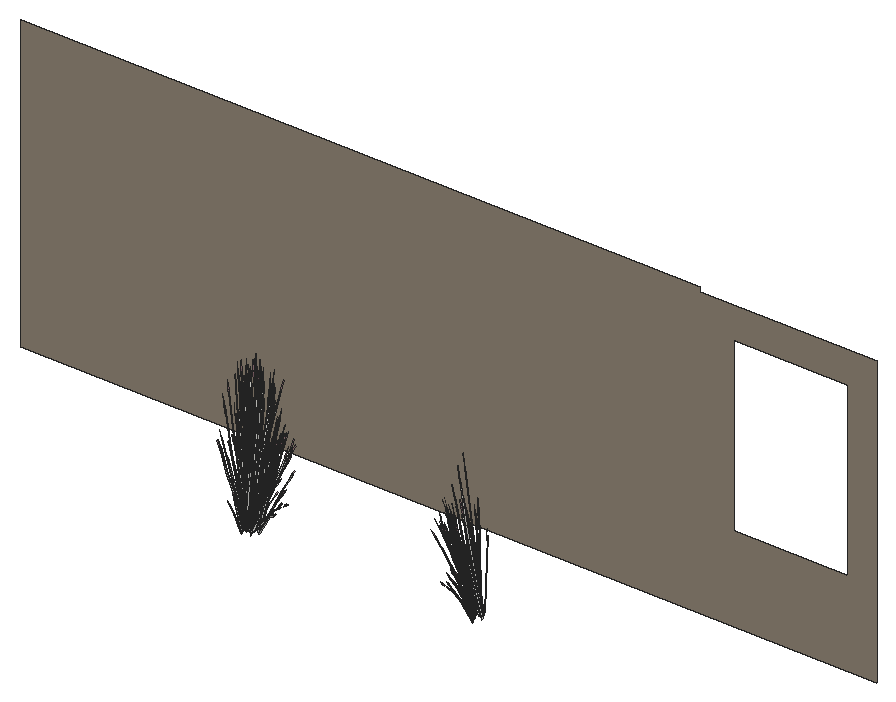
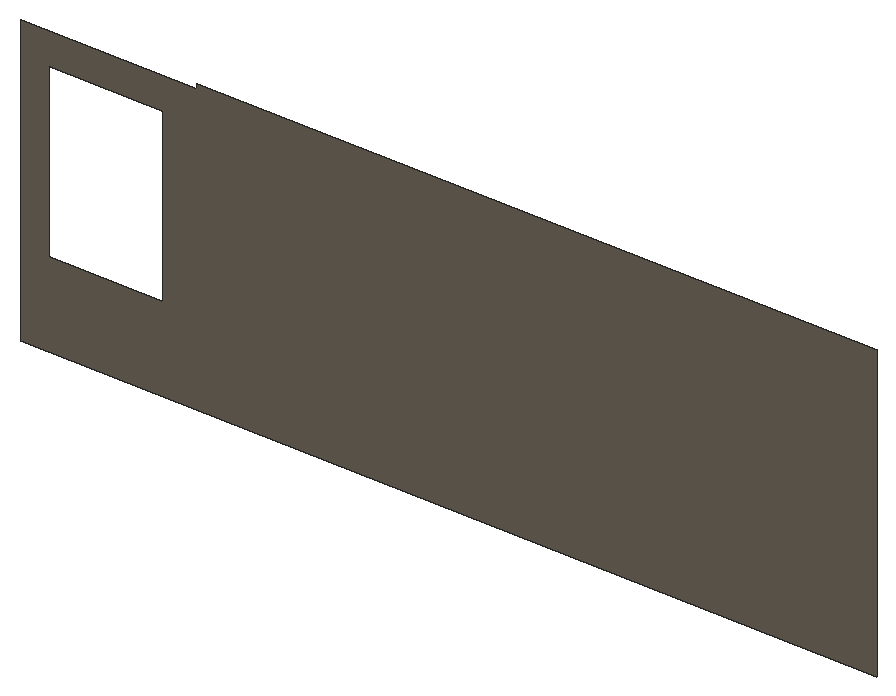
# SketchUp Ruby script. Lengths in inches.
U = 1.inch
M = Sketchup.active_model
def pt(a) = Geom::Point3d.new(a.map { |v| v * U })
def face(e, loops, mat)
  f = e.add_face(loops[0].map { |a| pt(a) })
  loops[1..].each { |l| e.add_face(l.map { |a| pt(a) }).erase! }
  f.material = f.back_material = mat if mat
  f
end
# faces: each face lists its corners as indices into pts; further lists are holes
def faces(e, pts, list, mat = nil) = list.each { |f| face(e, (f[0].is_a?(Array) ? f : [f]).map { |l| l.map { |i| pts[i] } }, mat) }
# xy, xz, yz: faces in a plane at the given z, y or x. An outline is a flat list of corners, or four numbers for a rectangle; further outlines are holes
def ring(l) = l.size == 4 ? [[l[0], l[1]], [l[2], l[1]], [l[2], l[3]], [l[0], l[3]]] : l.each_slice(2).to_a
def flat(e, list, mat, &to3) = list.each { |f| face(e, (f[0].is_a?(Array) ? f : [f]).map { |l| ring(l).map { |u, v| to3.(u, v) } }, mat) }
def xy(e, z, list, mat = nil) = flat(e, list, mat) { |x, y| [x, y, z] }
def xz(e, y, list, mat = nil) = flat(e, list, mat) { |x, z| [x, y, z] }
def yz(e, x, list, mat = nil) = flat(e, list, mat) { |y, z| [x, y, z] }
def lines(e, pts, list) = list.each { |a, b| e.add_line(pt(pts[a]), pt(pts[b])) }
# prism: a flat outline (further loops are holes) pulled along v
def prism(e, loops, v, mat = nil)
  f = face(e, loops, mat); d = Geom::Vector3d.new(v.map { |x| x * U })
  f.pushpull(f.normal.samedirection?(d) ? d.length : -d.length)
end
def box(e, o, s, mat = nil) = prism(e, [[o, [o[0] + s[0], o[1], o[2]], [o[0] + s[0], o[1] + s[1], o[2]], [o[0], o[1] + s[1], o[2]]]], [0, 0, s[2]], mat)
def at(x, y, z, deg = 0) = Geom::Transformation.translation(pt([x, y, z])) * Geom::Transformation.rotation(ORIGIN, Z_AXIS, deg.degrees)
def axes(o, x, y, z) = Geom::Transformation.new([*x, 0, *y, 0, *z, 0, *pt(o).to_a, 1])
def part(name) = M.definitions.add(name)
# library, detail: a bought-in or finely detailed component or shape, given as its bounding box
def library(name, o, s) = part(name).tap { |d| box(d.entities, o, s) }
def detail(e, o, s) = box(e.add_group.entities, o, s)
def put(e, d, t, mat = nil) = e.add_instance(d, t).tap { |i| i.material = mat if mat }
def group(e, t, mat = nil) = e.add_group.tap { |g| g.transformation = t; g.material = mat if mat }.entities
root = M.entities
M.materials.add("LightPink_Translucent").color = [144, 107, 117]
M.materials["LightPink_Translucent"].alpha = 0.75
M.materials.add("Plaster_04_1K").color = [142, 132, 117]
c1 = part("blade")
p = [[2.15,0.21,22],[0,0.17,0],[0.09,0.45,0],[2.18,0.31,22],[2.29,0.31,22],[0.38,0.45,0],
  [2.48,0.24,33],[2.49,0.24,33],[2.48,0.22,33]]
faces(c1.entities,p,[[0,1,2,3],[4,5,2,3],[6,3,4,7],[8,0,3,6]])
c2 = part("seeds")
p = [[0.3,-0.1,1.38],[-0.01,-0.03,1.59],[-0.01,-0.03,0.03],[0.14,-0.07,-0.07],[0.29,-0.03,3],[0.15,0.01,3.11]]
faces(c2.entities,p,[[0,1,2,3],[1,0,4,5]],"LightPink_Translucent")
c3 = part("blade with seeds")
put(c3.entities,c1,at(0,0,0))
put(c3.entities,c2,axes([2.4,0.25,30.99],[1.5799,-0.05474,1.17369],[-0.12525,1.92788,0.29478],[-0.07173,-0.02425,1.56792]))
xz(root,63.98,[[[48,-6,408,-6,408,114.97,333.82,114.97,333.82,117,48,117],[348,30,396,102]]],"Plaster_04_1K")
put(root,c3,axes([182.11,13.09,-3.52],[0,0.61104,0.49651],[-0.85008,0,0],[0,-0.13917,1.57504]))
put(root,c3,axes([186,15.4,-3.81],[-0.46912,-0.61443,-0.05142],[0.79476,-0.34146,0.51607],[-0.19584,0.0585,1.6363]))
put(root,c3,axes([182.99,15.125,-1],[0.54391,0.41056,-0.5672],[-0.57458,0.35956,-0.43934],[-0.08276,0.2086,1.08528]))
put(root,c3,axes([185.79,15.32,-3.97],[-0.70886,-0.15119,-0.30978],[0.17848,-0.53243,0.30978],[-0.1429,0.0614,1.38974]))
put(root,c3,axes([182.75,14.82,-0.95],[0.5141,-0.32171,0.35414],[0.48666,0.36734,-0.4572],[-0.07405,0.18664,0.87481]))
put(root,c3,axes([183.97,13.23,-3.33],[-0.85568,-0.29155,-0.29095],[0.41201,-0.61537,-0.50002],[-0.02689,-0.15109,1.59708]))
put(root,c3,axes([186.19,13.05,-3.16],[-0.02076,-0.57531,1.41272],[0.93937,0.14913,0.59816],[-0.22217,0.31481,1.3335]))
put(root,c3,axes([182.42,14.91,-0.6],[0.83505,0.03027,-0.13498],[-0.02282,0.57322,-0.74919],[-0.05801,0.22077,1.13838]))
put(root,c3,axes([182.4,15.74,-3.18],[0.69024,-0.1082,0.06507],[0.15868,0.43593,-0.86304],[-0.04376,0.22067,0.7736]))
put(root,c3,axes([185.67,13.78,-3.33],[0.08854,0.69723,-0.29095],[-0.92215,0.04216,-0.50002],[-0.16238,0.09287,1.59708]))
put(root,c3,axes([183.58,12.61,-3.9],[-0.31203,-0.62659,-0.69835],[0.89884,-0.22566,-0.18329],[-0.03449,-0.21218,1.54149]))
put(root,c3,axes([185.625,10.62,-0.97],[-0.74352,0.28449,-0.1216],[-0.36538,-0.50492,-0.67495],[-0.0981,-0.21277,1.02557]))
put(root,c3,axes([184.99,10.64,-1.32],[-0.7469,-0.15318,-0.51099],[0.25601,-0.52518,-0.3958],[-0.06849,-0.21144,0.97773]))
put(root,c3,axes([183.61,14.54,-2.125],[-0.0186,-0.23452,1.71376],[0.80601,0.15558,0.13857],[-0.04985,0.33422,0.73262]))
put(root,c3,axes([182.11,12.54,-3.97],[0.53038,-0.38124,-0.30978],[0.53038,0.38124,0.30978],[0,-0.1228,1.38974]))
put(root,c3,axes([184.5,10.07,-3.87],[-0.52505,0.35054,-0.03893],[-0.48109,-0.38392,-0.17649],[-0.03387,-0.10878,0.58215]))
put(root,c3,axes([184.29,13.53,-3.64],[0.96033,0.12874,0.45755],[-0.19544,0.7271,0.17955],[-0.14034,-0.07021,1.58856]))
put(root,c3,axes([184.04,13.4,-3.28],[-0.36864,0.55059,0.44739],[-0.76598,-0.26498,-0.21531],[0,-0.12692,1.43643]))
put(root,c3,axes([185.26,10.74,-1.02],[-0.36264,-0.49684,-0.71045],[0.74649,-0.27689,0.08574],[-0.0848,-0.24006,1.00501]))
put(root,c3,axes([183.78,14.6875,-3.53],[0.81646,-0.16218,0.17642],[0.20161,0.60355,0.35086],[-0.07282,-0.08794,1.60407]))
put(root,c3,axes([184.83,14.78,-3.8],[-0.76598,-0.27433,0],[0.36864,-0.57001,0],[0,0,1.62707]))
put(root,c3,axes([185.4,10.82,-0.95],[-0.22906,0.4699,0.35414],[-0.66828,-0.13705,-0.4572],[-0.06128,-0.18919,0.87481]))
put(root,c3,axes([186.6,15.47,-3.625],[0.47504,0.61229,0],[-0.79476,0.34146,-0.51607],[-0.18101,0.07777,1.63711]))
put(root,c3,axes([184.18,15.73,-0.9375],[-0.74868,-0.15974,0.53283],[0.25601,-0.52518,0.43934],[0.04499,0.20653,1.10256]))
put(root,c3,axes([183.98,15.77,-1.27],[-0.55987,0.20767,0.0643],[-0.27403,-0.37869,0.50621],[0.05407,0.16693,0.77189]))
put(root,c3,axes([186.21,14.72,-3.53],[0.21949,-0.60727,0.17642],[0.8032,0.17185,0.35086],[-0.13875,0.00296,1.60407]))
put(root,c3,axes([185.83,13.92,-3.38],[0.56134,0.36712,0.1448],[-0.46823,0.41419,-0.41347],[-0.13033,0.05599,1.26744]))
put(root,c3,axes([185.64,13.46,-3.7],[-0.70674,-0.52593,-0.06131],[0.70717,-0.52625,0],[-0.02468,-0.01837,1.75571]))
put(root,c3,axes([185.82,13.65,-3.28],[0.82508,-0.03772,0.44739],[0.07462,0.62614,-0.21531],[-0.14771,0.06346,1.43643]))
put(root,c3,axes([186.02,15.09,-3.67],[0.95122,0.19861,0.30756],[-0.23797,0.7099,-0.36492],[-0.15744,0.08885,1.64885]))
put(root,c3,axes([184.63,9.64,-4.51],[-0.12744,0.02202,1.76342],[-0.70477,-0.24781,-0.26939],[0.01183,-0.2067,0.30037]))
put(root,c3,axes([186.43,15.05,-3.52],[0.7111,-0.30552,0.49651],[0.42504,0.54784,0],[-0.16196,0.06958,1.57504]))
put(root,c3,axes([185.33,10.32,-1.47],[0.22906,-0.4699,-0.35414],[0.66828,0.13705,0.4572],[-0.06128,-0.18919,0.87481]))
put(root,c3,axes([184.21,12.86,-3.64],[0.33034,0.68327,0.45755],[-0.94388,0.2376,0.17955],[0.01154,-0.12555,1.58856]))
put(root,c3,axes([184.06,12.77,-3.79],[0.36864,-0.55059,-0.44739],[0.76598,0.26498,0.21531],[0,-0.12692,1.43643]))
put(root,c3,axes([185,14.55,-3.8],[-0.24791,-0.5268,0],[0.70791,-0.18448,0],[0,0,1.54371]))
put(root,c3,axes([184.1,15.66,-4.51],[0.12297,-0.03325,1.76342],[0.73967,0.18301,-0.26939],[0.02163,0.20626,0.30037]))
put(root,c3,axes([184.26,15.84,-1.47],[-0.22906,0.4699,-0.35414],[-0.66828,-0.13705,0.4572],[0.06128,0.18919,0.87481]))
put(root,c3,axes([186,13.51,-3.79],[-0.36864,0.55059,-0.44739],[-0.76598,-0.26498,0.21531],[0,0.12692,1.43643]))
put(root,c3,axes([185.61,10.39,-1.27],[0.55987,-0.20767,0.0643],[0.27403,0.37869,0.50621],[-0.05407,-0.16693,0.77189]))
put(root,c3,axes([183.79,16.68,-1.28],[0.09631,0.0984,1.74944],[0.77725,0.03866,-0.27667],[0.07816,0.217,0.14031]))
put(root,c3,axes([187.46,13.17,-3.53],[-0.59697,-0.44509,0.17642],[0.60159,-0.4317,0.35086],[-0.06593,0.0909,1.60407]))
put(root,c3,axes([185.4,12.92,-3.79],[0,-0.70701,0],[0.95008,0,0],[0,0,1.79456]))
put(root,c3,axes([185.41,10.43,-1.27],[0.74868,0.15974,0.48003],[-0.25601,0.52518,0.3958],[-0.04499,-0.20653,0.9933]))
put(root,c3,axes([184.51,13.04,-3.57],[0.8561,0.29616,0.24065],[-0.41201,0.61537,0.50002],[0,-0.14185,1.60543]))
put(root,c3,axes([185.875,13.2,-3.71],[0,0.70667,-0.05637],[-0.95008,0,0],[0,0.02221,1.79368]))
put(root,c3,axes([184.24,12.63,-3.28],[-0.82508,0.03772,0.44739],[-0.07462,-0.62614,-0.21531],[0.14771,-0.06346,1.43643]))
put(root,c3,axes([184.19,15.35,-0.95],[0.22906,-0.4699,0.35414],[0.66828,0.13705,-0.4572],[0.06128,0.18919,0.87481]))
put(root,c3,axes([183.85,11.56,-3.53],[-0.21949,0.60727,0.17642],[-0.8032,-0.17185,0.35086],[0.13875,-0.00296,1.60407]))
put(root,c3,axes([185.42,14.57,-3.71],[0.33034,0.70197,-0.06012],[-0.94388,0.24598,0],[0.01154,0.02451,1.72173]))
put(root,c3,axes([183.46,10.81,-3.625],[-0.47504,-0.61229,0],[0.79476,-0.34146,-0.51607],[0.18101,-0.07777,1.63711]))
put(root,c3,axes([184.33,15.42,-1.02],[0.36264,0.49684,-0.71045],[-0.74649,0.27689,0.08574],[0.0848,0.24006,1.00501]))
put(root,c3,axes([188.15,13.64,-3.8],[-0.94962,-0.00489,-0.04976],[0,-0.68292,0.49943],[-0.02984,0.15546,1.58352]))
put(root,c3,axes([186.28,11.59,-3.53],[-0.81646,0.16218,0.17642],[-0.20161,-0.60355,0.35086],[0.07282,0.08794,1.60407]))
put(root,c3,axes([185.45,9.33,-3.23],[0.09747,0.35631,1.1486],[-0.54071,-0.19735,0.84392],[0.05818,-0.18244,0.25299]))
put(root,c3,axes([185.09,17.03,-0.35],[0.52505,-0.35054,-0.06488],[0.48109,0.38392,-0.29416],[0.03387,0.10878,0.97024]))
put(root,c3,axes([184.95,12.47,-3.64],[-0.62999,0.55453,0.45755],[-0.74845,-0.4895,0.17955],[0.15188,-0.05534,1.58856]))
put(root,c3,axes([186.02,13.34,-3.79],[0.53038,0.39469,0],[-0.53038,0.39469,0],[0,0,1.69266]))
put(root,c3,axes([186.02,12.88,-3.28],[0.36864,-0.55059,0.44739],[0.76598,0.26498,-0.21531],[0,0.12692,1.43643]))
put(root,c3,axes([185.7,14.8,-3.8],[0.76598,0.27433,0],[-0.36864,0.57001,0],[0,0,1.74954]))
put(root,c3,axes([184.6,15.52,-1.32],[0.7469,0.15318,-0.51099],[-0.25601,0.52518,-0.3958],[0.06849,0.21144,0.97773]))
put(root,c3,axes([183.97,15.55,-0.97],[0.74352,-0.28449,-0.1216],[0.36538,0.50492,-0.67495],[0.0981,0.21277,1.02557]))
put(root,c3,axes([185.77,12.75,-3.62],[-0.96033,-0.12874,0.49198],[0.19544,-0.7271,0.19306],[0.14034,0.07021,1.70813]))
put(root,c3,axes([187.76,9.91,-1.29],[-0.07716,0.04667,1.77383],[-0.75601,-0.15746,-0.16761],[-0.02737,-0.20368,0.31391]))
put(root,c3,axes([187.17,11.26,-0.97],[-0.83505,-0.03027,-0.1216],[0.02282,-0.57322,-0.67495],[0.05801,-0.22077,1.02557]))
put(root,c3,axes([187.95,13.74,-3.97],[-0.53038,0.38124,-0.30978],[-0.53038,-0.38124,0.30978],[0,0.1228,1.38974]))
put(root,c3,axes([186.4375,13.67,-3.91],[0.2786,0.55945,-0.69212],[-0.80253,0.20149,-0.18165],[0.03079,0.18945,1.52773]))
put(root,c3,axes([186.04,13.07,-3.79],[0.85008,0,0],[0,0.63259,0],[0,0,1.78407]))
put(root,c3,axes([186.84,11.35,-0.95],[-0.5141,0.32171,0.35414],[-0.48666,-0.36734,-0.4572],[0.07405,-0.18664,0.87481]))
put(root,c3,axes([185.22,12.375,-3.28],[-0.45644,-0.51287,0.44739],[0.69137,-0.36116,-0.21531],[0.14771,0.06346,1.43643]))
put(root,c3,axes([184.39,12.5,-3.33],[-0.08854,-0.69723,-0.29095],[0.92215,-0.04216,-0.50002],[0.16238,-0.09287,1.59708]))
put(root,c3,axes([186.34,13.01,-3.38],[0.70791,-0.1782,0.1448],[0.24791,0.50885,-0.41347],[0,0.11199,1.26744]))
put(root,c3,axes([186.6,11.04,-1.32],[-0.54391,-0.41056,-0.51099],[0.57458,-0.35956,-0.3958],[0.08276,-0.2086,0.97773]))
put(root,c3,axes([186.09,13.05,-3.33],[0.85568,0.29155,-0.29095],[-0.41201,0.61537,-0.50002],[0.02689,0.15109,1.59708]))
put(root,c3,axes([184.27,10.95,-3.97],[0.70886,0.15119,-0.30978],[-0.17848,0.53243,0.30978],[0.1429,-0.0614,1.38974]))
put(root,c3,axes([186.24,10.3125,-3.41],[-0.21597,0.12368,1.43002],[-0.64681,-0.21647,-0.30754],[0.1199,-0.26922,0.61141]))
put(root,c3,axes([187.95,13.19,-3.52],[0,-0.61104,0.49651],[0.85008,0,0],[0,0.13917,1.57504]))
put(root,c3,axes([188.32,13.76,-3.98],[0,0.61104,-0.49651],[-0.85008,0,0],[0,0.13917,1.57504]))
put(root,c3,axes([186.05,15.61,-1.27],[-0.75571,0.14023,0.48003],[-0.13115,-0.55007,0.3958],[0.17773,0.16212,0.9933]))
put(root,c3,axes([184.11,10.71,-3.98],[0.7111,-0.30552,-0.49651],[0.42504,0.54784,0],[0.16196,-0.06958,1.57504]))
put(root,c3,axes([185.9,15.72,-1.27],[-0.34533,0.38816,0.0643],[-0.49176,-0.22599,0.50621],[0.15898,0.12445,0.77189]))
put(root,c3,axes([185.03,14.4375,-2.125],[-0.17368,-0.19618,1.71376],[0.80256,-0.16516,0.13857],[0.18139,0.30799,0.73262]))
put(root,c3,axes([185.53,12.23,-3.38],[0.14658,-0.54532,0.1448],[0.71613,0.09466,-0.41347],[0.13033,0.05599,1.26744]))
put(root,c3,axes([186.55,11.28,-3.52],[-0.7111,-0.30552,0.49651],[0.42504,-0.54784,0],[0.16196,0.06958,1.57504]))
put(root,c3,axes([186.77,11.23,-1.02],[0.01977,-0.56521,-0.71045],[0.83252,0.03796,0.08574],[0.08786,-0.23945,1.00501]))
put(root,c3,axes([185.93,14.47,-3.82],[0.79769,-0.20732,-0.19198],[0.2803,0.59721,0.00008],[0.08805,-0.02292,1.73897]))
put(root,c3,axes([185.79,15.27,-0.95],[-0.11735,-0.49217,0.35414],[0.67083,-0.12996,-0.4572],[0.18018,0.14104,0.87481]))
put(root,c3,axes([185.94,12.7,-3.79],[0.45644,0.51287,-0.44739],[-0.69137,0.36116,0.21531],[0.14771,0.06346,1.43643]))
put(root,c3,axes([186.25,12.44,-1.53],[-0.65655,-0.31748,1.38283],[0.69326,-0.49431,0.59665],[0.21183,0.29789,1.33663]))
put(root,c3,axes([187.11,10.89,-1.47],[0.5141,-0.32171,-0.35414],[0.48666,0.36734,0.4572],[0.07405,-0.18664,0.87481]))
put(root,c3,axes([185.14,15.96,-1.29],[0.00225,-0.07398,1.77383],[0.65113,-0.32638,-0.16761],[0.22617,0.1165,0.31391]))
put(root,c3,axes([187.31,11.05,-1.27],[0.62439,0.02847,0.0643],[-0.01712,0.42991,0.50621],[0.06534,-0.16468,0.77189]))
put(root,c3,axes([187.24,15.02,-3.23],[-0.4278,-0.1757,1.1486],[0.5524,-0.17852,0.84392],[0.14899,0.15122,0.25299]))
put(root,c3,axes([185.71,14.84,-3.41],[0.01341,-0.20255,1.43002],[0.64074,-0.22625,-0.30754],[0.1978,0.24243,0.61141]))
put(root,c3,axes([187.93,10.35,-1.28],[-0.00733,-0.12161,1.74944],[-0.61946,-0.35147,-0.27667],[0.09577,-0.21306,0.14031]))
put(root,c3,axes([184.95,11.97,-3.94],[0.51177,-0.45928,-0.62353],[0.63575,0.41646,-0.16365],[0.20507,-0.11457,1.37633]))
put(root,c3,axes([187.11,11.01,-1.27],[0.54105,0.41691,0.48003],[-0.57458,0.35956,0.3958],[0.0998,-0.1956,0.9933]))
put(root,c3,axes([187.19,11.56,-3.97],[0.17848,0.53243,-0.30978],[-0.70886,0.15119,0.30978],[0.1429,0.0614,1.38974]))
put(root,c3,axes([188.53,13.29,-3.625],[0.95008,0,0],[0,0.68292,-0.51607],[0,0.15554,1.63711]))
put(root,c3,axes([185.46,12.41,-3.33],[0.76714,-0.40567,-0.29095],[0.51013,0.57321,-0.50002],[0.18927,0.05821,1.59708]))
put(root,c3,axes([187.3,15.82,-3.33],[-0.48723,-0.01916,1.0506],[0.32177,-0.40701,0.58006],[0.19248,0.1446,0.8241]))
put(root,c3,axes([187.74,12.34,-0.95],[-0.66138,0.08733,0.35414],[-0.17464,-0.49921,-0.4572],[0.18953,-0.13408,0.87481]))
put(root,c3,axes([185.83,10.94,-2.125],[-0.14147,0.21002,1.71376],[-0.59349,-0.43464,0.13857],[0.26773,-0.27089,0.73262]))
put(root,c3,axes([185.73,15.53,-0.97],[0.45276,-0.52302,-0.1216],[0.65568,0.30132,-0.67495],[0.22792,0.14777,1.02557]))
put(root,c3,axes([183.52,12.05,-4.41],[-0.74787,0.24464,1.28929],[-0.23804,-0.70192,0.50096],[0.45924,0.01168,1.46642]))
put(root,c3,axes([188.08,12.39,-0.97],[-0.70283,-0.33692,-0.1216],[0.40491,-0.48793,-0.67495],[0.19857,-0.16961,1.02557]))
put(root,c3,axes([186.27,15.27,-1.32],[0.74975,-0.14525,-0.51099],[0.13115,0.55007,-0.3958],[0.20138,0.15763,0.97773]))
put(root,c3,axes([186.96,10.96,-3.625],[0.47504,-0.61229,0],[0.79476,0.34146,-0.51607],[0.18101,0.07777,1.63711]))
put(root,c3,axes([187.75,10.69,-4.51],[-0.11372,-0.04814,1.76342],[-0.29211,-0.53779,-0.26939],[0.19706,-0.14594,0.30037]))
put(root,c3,axes([187.13,14.61,-0.95],[-0.43232,-0.38257,0.35414],[0.49364,-0.36215,-0.4572],[0.25081,0.0551,0.87481]))
put(root,c3,axes([187.39,11.33,-3.98],[0.7111,0.30552,-0.49651],[-0.42504,0.54784,0],[0.16196,0.06958,1.57504]))
put(root,c3,axes([187.52,14.95,-1.27],[-0.03826,0.46465,0.0643],[-0.57772,-0.01274,0.50621],[0.2213,0.04862,0.77189]))
put(root,c3,axes([187.36,15.68,-4.51],[0.05536,-0.08822,1.76342],[0.69692,-0.25981,-0.26939],[0.21129,0.13447,0.30037]))
put(root,c3,axes([187.58,14.81,-1.27],[-0.56024,0.40262,0.48003],[-0.48318,-0.42758,0.3958],[0.26285,0.07427,0.9933]))
put(root,c3,axes([187.73,11.99,-1.32],[-0.19519,-0.55794,-0.51099],[0.73919,-0.0976,-0.3958],[0.21183,-0.14986,0.97773]))
put(root,c3,axes([189.03,14.87,-2.07],[-0.14542,-0.51365,-0.03492],[0.68734,-0.11809,-0.15832],[0.14353,0.03256,0.52218]))
put(root,c3,axes([187.84,13.53,-0.95],[-0.63144,-0.17046,0.35414],[0.18417,-0.49731,-0.4572],[0.25423,-0.0456,0.87481]))
put(root,c3,axes([186.35,12.5,-3.94],[0.79037,0.10018,-0.62353],[-0.16679,0.61794,-0.16365],[0.23587,0.07488,1.37633]))
put(root,c3,axes([189.72,12.86,-3.74],[-0.47106,-0.39072,-0.06488],[0.51591,-0.35801,-0.29416],[0.14618,-0.02521,0.97024]))
put(root,c3,axes([188.64,10.875,-3.23],[-0.25308,0.31105,1.1486],[-0.21753,-0.4179,0.84392],[0.20902,-0.10472,0.25299]))
put(root,c3,axes([188.34,12.26,-1.27],[0.52161,0.25698,0.0643],[-0.30368,0.36595,0.50621],[0.16723,-0.11831,0.77189]))
put(root,c3,axes([188.19,12.15,-1.27],[0.18844,0.56237,0.48003],[-0.73919,0.0976,0.3958],[0.21785,-0.13226,0.9933]))
put(root,c3,axes([186.19,13.83,-2.125],[-0.28223,-0.10528,1.71376],[0.58406,-0.44165,0.13857],[0.36402,0.19924,0.73262]))
put(root,c3,axes([189.81,12.24,-1.29],[-0.09924,-0.00464,1.77383],[-0.4121,-0.49725,-0.16761],[0.1655,-0.1635,0.31391]))
put(root,c3,axes([188.28,12.04,-1.47],[0.66138,-0.08733,-0.35414],[0.17464,0.49921,0.4572],[0.18953,-0.13408,0.87481]))
put(root,c3,axes([187.75,12.21,-1.02],[0.39688,-0.48213,-0.71045],[0.69548,0.34264,0.08574],[0.23697,-0.17468,1.00501]))
put(root,c3,axes([188.41,13.6875,-1.27],[0.27906,0.41663,0.0643],[-0.50888,0.20393,0.50621],[0.22432,-0.04024,0.77189]))
put(root,c3,axes([187.74,14.81,-1.47],[0.43232,0.38257,-0.35414],[-0.49364,0.36215,0.4572],[0.25081,0.0551,0.87481]))
put(root,c3,axes([187.25,14.85,-0.97],[0.04068,-0.62141,-0.1216],[0.77029,0.01698,-0.67495],[0.29667,0.04317,1.02557]))
put(root,c3,axes([188.11,13.7,-0.97],[-0.38229,-0.5533,-0.1216],[0.6785,-0.2719,-0.67495],[0.28593,-0.073,1.02557]))
put(root,c3,axes([188.36,13.54,-1.27],[-0.21466,0.55714,0.48003],[-0.70573,-0.19051,0.3958],[0.27753,-0.03348,0.9933]))
put(root,c3,axes([187.92,14.48,-1.28],[0.16299,-0.01033,1.74944],[0.44707,-0.47471,-0.27667],[0.28992,0.06266,0.14031]))
put(root,c3,axes([188.07,13.22,-1.32],[0.20584,-0.55581,-0.51099],[0.70573,0.19051,-0.3958],[0.28414,-0.05097,0.97773]))
put(root,c3,axes([189.85,13.58,-3.23],[-0.46945,0.10088,1.1486],[0.22097,-0.4169,0.84392],[0.24904,0.02853,0.25299]))
put(root,c3,axes([188.33,11.77,-3.41],[-0.27143,-0.0181,1.43002],[-0.27808,-0.48551,-0.30754],[0.33346,-0.13735,0.61141]))
put(root,c3,axes([188.51,13.48,-1.47],[0.63144,0.17046,-0.35414],[-0.18417,0.49731,0.4572],[0.25423,-0.0456,0.87481]))
put(root,c3,axes([187.29,14.55,-1.02],[0.75952,0.01471,-0.71045],[-0.05101,0.61953,0.08574],[0.32177,0.06538,1.00501]))
put(root,c3,axes([188.83,13.38,-4.02],[-0.48937,0.07333,1.41583],[-0.07789,-0.58369,0.08104],[0.34275,-0.08835,0.80566]))
put(root,c3,axes([189.36,13,-4.51],[-0.03971,-0.09277,1.76342],[0.27541,-0.54264,-0.26939],[0.27782,-0.00781,0.30037]))
put(root,c3,axes([189.63,15.34,-1.29],[-0.0687,-0.05349,1.77383],[0.15029,-0.57341,-0.16761],[0.27062,-0.03664,0.31391]))
put(root,c3,axes([186.79,12.86,-2.125],[-0.31515,0.01384,1.71376],[0.20907,-0.5998,0.13857],[0.44912,0.0371,0.73262]))
put(root,c3,axes([187.94,13.43,-1.02],[0.66765,-0.26986,-0.71045],[0.37208,0.55551,0.08574],[0.32259,-0.0631,1.00501]))
put(root,c3,axes([190.18,12.83,-1.28],[0.10543,-0.09307,1.74944],[-0.13495,-0.57092,-0.27667],[0.26455,-0.10825,0.14031]))
put(root,c3,axes([188.97,14.25,-3.41],[-0.18299,-0.15028,1.43002],[0.23809,-0.49714,-0.30754],[0.37023,0.06735,0.61141]))
put(root,c3,axes([280.36,12.17,-2.125],[0.31515,-0.01384,1.71376],[-0.20907,0.5998,0.13857],[-0.44912,-0.0371,0.73262]))
put(root,c3,axes([280.49,13.23,-2.125],[0.26363,-0.12925,1.71376],[0.22195,0.59723,0.13857],[-0.41388,0.13498,0.73262]))
put(root,c3,axes([279.67,14.24,-3.41],[0.26405,0.05016,1.43002],[0.17019,0.51235,-0.30754],[-0.35868,0.0959,0.61141]))
put(root,c3,axes([282,12.6,-2.66],[0.21597,-0.08839,1.77064],[0.07448,0.61717,0.13857],[-0.4678,0.08189,0.63284]))
put(root,c3,axes([279.68,13.02,-1.28],[-0.12407,0.07933,1.74944],[0.01055,0.57963,-0.27667],[-0.2844,0.07538,0.14031]))
put(root,c3,axes([281.3,11.61,-1.02],[-0.75952,-0.01471,-0.71045],[0.05101,-0.61953,0.08574],[-0.32177,-0.06538,1.00501]))
put(root,c3,axes([280.6875,11.76,-3.41],[0.14835,0.17012,1.43002],[-0.34183,0.46242,-0.30754],[-0.351,-0.11053,0.61141]))
put(root,c3,axes([280.08,12.6875,-1.47],[-0.63144,-0.17046,-0.35414],[0.18417,-0.49731,0.4572],[-0.25423,0.0456,0.87481]))
put(root,c3,axes([280.95,11.21,-2.125],[0.28223,0.10528,1.71376],[-0.58406,0.44165,0.13857],[-0.36402,-0.19924,0.73262]))
put(root,c3,axes([278.3,13.6,-1.29],[0.09697,0.01639,1.77383],[0.29997,0.53988,-0.16761],[-0.1985,0.1417,0.31391]))
put(root,c3,axes([280.51,12.94,-1.32],[-0.20584,0.55581,-0.51099],[-0.70573,-0.19051,-0.3958],[-0.28414,0.05097,0.97773]))
put(root,c3,axes([281.05,11.74,-1.32],[-0.55171,0.40476,-0.51099],[-0.48318,-0.42758,-0.3958],[-0.28031,-0.06159,0.97773]))
put(root,c3,axes([280.16,12.91,-4.51],[0.01927,0.0963,1.76342],[-0.38846,0.5029,-0.26939],[-0.27592,-0.02535,0.30037]))
put(root,c3,axes([280.27,10.6,-1.29],[0.05633,0.06098,1.77383],[-0.27155,0.54815,-0.16761],[-0.27501,0.00397,0.31391]))
put(root,c3,axes([279.12,15.32,-3.23],[0.31665,-0.27694,1.1486],[0.12495,0.43841,0.84392],[-0.22883,0.0785,0.25299]))
put(root,c3,axes([280.9,10.24,-1.28],[-0.16348,-0.00431,1.74944],[-0.52047,0.43131,-0.27667],[-0.2777,-0.08813,0.14031]))
put(root,c3,axes([280.23,12.625,-1.27],[0.21466,-0.55714,0.48003],[0.70573,0.19051,0.3958],[-0.27753,0.03348,0.9933]))
put(root,c3,axes([280.48,12.46,-0.97],[0.38229,0.5533,-0.1216],[-0.6785,0.2719,-0.67495],[-0.28593,0.073,1.02557]))
put(root,c3,axes([281.34,11.32,-0.97],[-0.04068,0.62141,-0.1216],[-0.77029,-0.01698,-0.67495],[-0.29667,-0.04317,1.02557]))
put(root,c3,axes([280.84,11.36,-1.47],[-0.43232,-0.38257,-0.35414],[0.49364,-0.36215,0.4572],[-0.25081,-0.0551,0.87481]))
put(root,c3,axes([280.17,12.48,-1.27],[-0.27906,-0.41663,0.0643],[0.50888,-0.20393,0.50621],[-0.22432,0.04024,0.77189]))
put(root,c3,axes([281.45,13.63,-2.125],[0.18977,-0.18775,1.71376],[0.47917,0.50677,0.13857],[-0.32866,0.23079,0.73262]))
put(root,c3,axes([280.3125,14.12,-1.47],[-0.66138,0.08733,-0.35414],[-0.17464,-0.49921,0.4572],[-0.18953,0.13408,0.87481]))
put(root,c3,axes([279.95,15.6,-4.51],[0.10192,0.06105,1.76342],[0.17281,0.56562,-0.26939],[-0.22588,0.12062,0.30037]))
put(root,c3,axes([279.81,12.28,-3.23],[0.48508,-0.04372,1.1486],[-0.3077,0.38525,0.84392],[-0.23971,-0.05779,0.25299]))
put(root,c3,axes([280.4,14.01,-1.27],[-0.18844,-0.56237,0.48003],[0.73919,-0.0976,0.3958],[-0.21785,0.13226,0.9933]))
put(root,c3,axes([280.78,11.21,-0.91],[0.62747,-0.45094,0.53763],[0.54116,0.47889,0.4433],[-0.29439,-0.08318,1.11249]))
put(root,c3,axes([280.25,13.9,-1.27],[-0.52161,-0.25698,0.0643],[0.30368,-0.36595,0.50621],[-0.16723,0.11831,0.77189]))
put(root,c3,axes([281.3125,14.09,-2.125],[0.14147,-0.21002,1.71376],[0.59349,0.43464,0.13857],[-0.26773,0.27089,0.73262]))
put(root,c3,axes([280.75,12.63,-0.95],[0.63144,0.17046,0.35414],[-0.18417,0.49731,-0.4572],[-0.25423,0.0456,0.87481]))
put(root,c3,axes([280.86,14.18,-1.32],[0.19519,0.55794,-0.51099],[-0.73919,0.0976,-0.3958],[-0.21183,0.14986,0.97773]))
put(root,c3,axes([281.07,11.21,-1.27],[0.03826,-0.46465,0.0643],[0.57772,0.01274,0.50621],[-0.2213,-0.04862,0.77189]))
put(root,c3,axes([279.7,15.18,-1.28],[-0.01889,0.12092,1.74944],[0.53598,0.42065,-0.27667],[-0.14032,0.19892,0.14031]))
put(root,c3,axes([282.7,13.78,-3.94],[-0.79037,-0.10018,-0.62353],[0.16679,-0.61794,-0.16365],[-0.23587,-0.07488,1.37633]))
put(root,c3,axes([282.84,10.41,-0.57],[-0.50709,0.58578,-0.13619],[-0.73436,-0.33748,-0.75594],[-0.25527,-0.1655,1.14864]))
put(root,c3,axes([281.46,11.56,-0.95],[0.43232,0.38257,0.35414],[-0.49364,0.36215,-0.4572],[-0.25081,-0.0551,0.87481]))
put(root,c3,axes([282.62,10.88,-1.02],[-0.64788,-0.29534,-0.71045],[0.46044,-0.51755,0.08574],[-0.23473,-0.17635,1.00501]))
put(root,c3,axes([282.32,10.9,-1.32],[-0.74975,0.14525,-0.51099],[-0.13115,-0.55007,-0.3958],[-0.20138,-0.15763,0.97773]))
put(root,c3,axes([281.66,14.95,-3.98],[-0.7111,-0.30552,-0.49651],[0.42504,-0.54784,0],[-0.16196,-0.06958,1.57504]))
put(root,c3,axes([281.35,10.4,-4.51],[-0.0736,0.08049,1.76342],[-0.74378,0.17355,-0.26939],[-0.17968,-0.15788,0.30037]))
put(root,c3,axes([280.51,13.78,-0.97],[0.70283,0.33692,-0.1216],[-0.40491,0.48793,-0.67495],[-0.19857,0.16961,1.02557]))
put(root,c3,axes([282.1,15.32,-3.625],[-0.47504,0.61229,0],[-0.79476,-0.34146,-0.51607],[-0.18101,-0.07777,1.63711]))
put(root,c3,axes([279.35,15.24,-0.35],[0.67048,0.16311,-0.06488],[-0.20625,0.50201,-0.29416],[-0.10966,0.07622,0.97024]))
put(root,c3,axes([280.85,13.83,-0.95],[0.66138,-0.08733,0.35414],[0.17464,0.49921,-0.4572],[-0.18953,0.13408,0.87481]))
put(root,c3,axes([281.23,16.2,-3.41],[0.23977,-0.09639,1.43002],[0.59198,0.29065,-0.30754],[-0.1762,0.25149,0.61141]))
put(root,c3,axes([280.89,10.71,-3.87],[-0.21918,0.49894,-0.03893],[-0.6746,-0.15348,-0.17649],[-0.10242,-0.08161,0.58215]))
put(root,c3,axes([282.65,9.02,-1.29],[-0.01417,0.07324,1.77383],[-0.6991,0.2658,-0.16761],[-0.20573,-0.13587,0.31391]))
